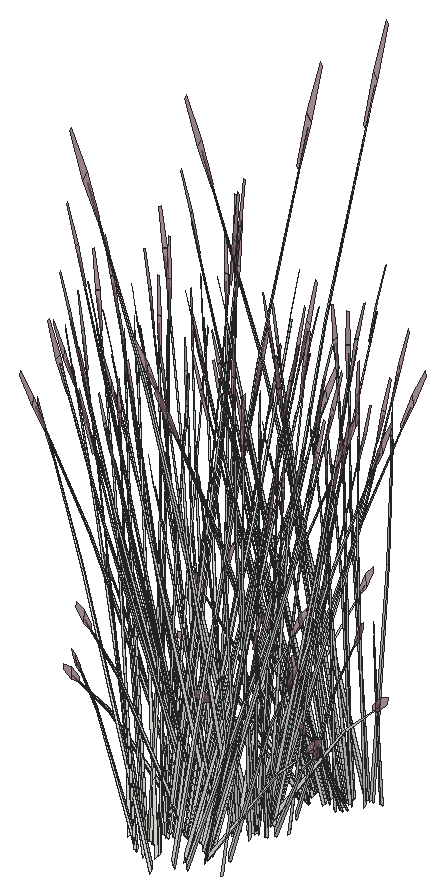
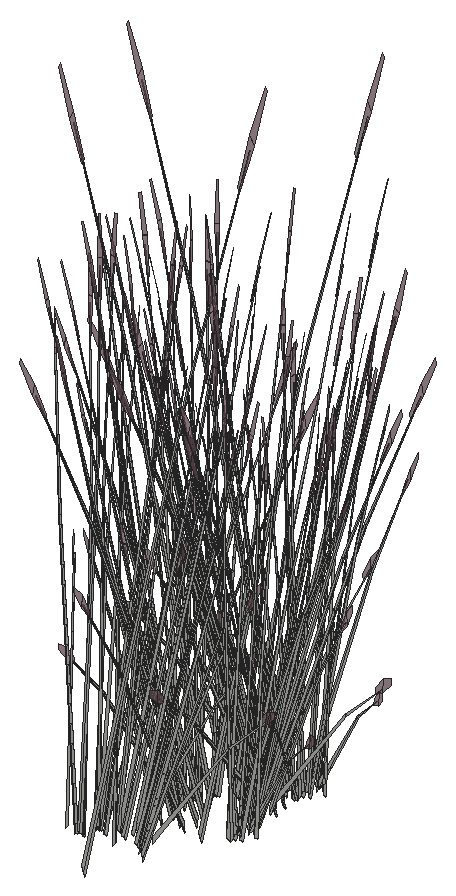
# SketchUp Ruby script. Lengths in inches.
U = 1.inch
M = Sketchup.active_model
def pt(a) = Geom::Point3d.new(a.map { |v| v * U })
def face(e, loops, mat)
  f = e.add_face(loops[0].map { |a| pt(a) })
  loops[1..].each { |l| e.add_face(l.map { |a| pt(a) }).erase! }
  f.material = f.back_material = mat if mat
  f
end
# faces: each face lists its corners as indices into pts; further lists are holes
def faces(e, pts, list, mat = nil) = list.each { |f| face(e, (f[0].is_a?(Array) ? f : [f]).map { |l| l.map { |i| pts[i] } }, mat) }
# xy, xz, yz: faces in a plane at the given z, y or x. An outline is a flat list of corners, or four numbers for a rectangle; further outlines are holes
def ring(l) = l.size == 4 ? [[l[0], l[1]], [l[2], l[1]], [l[2], l[3]], [l[0], l[3]]] : l.each_slice(2).to_a
def flat(e, list, mat, &to3) = list.each { |f| face(e, (f[0].is_a?(Array) ? f : [f]).map { |l| ring(l).map { |u, v| to3.(u, v) } }, mat) }
def xy(e, z, list, mat = nil) = flat(e, list, mat) { |x, y| [x, y, z] }
def xz(e, y, list, mat = nil) = flat(e, list, mat) { |x, z| [x, y, z] }
def yz(e, x, list, mat = nil) = flat(e, list, mat) { |y, z| [x, y, z] }
def lines(e, pts, list) = list.each { |a, b| e.add_line(pt(pts[a]), pt(pts[b])) }
# prism: a flat outline (further loops are holes) pulled along v
def prism(e, loops, v, mat = nil)
  f = face(e, loops, mat); d = Geom::Vector3d.new(v.map { |x| x * U })
  f.pushpull(f.normal.samedirection?(d) ? d.length : -d.length)
end
def box(e, o, s, mat = nil) = prism(e, [[o, [o[0] + s[0], o[1], o[2]], [o[0] + s[0], o[1] + s[1], o[2]], [o[0], o[1] + s[1], o[2]]]], [0, 0, s[2]], mat)
def at(x, y, z, deg = 0) = Geom::Transformation.translation(pt([x, y, z])) * Geom::Transformation.rotation(ORIGIN, Z_AXIS, deg.degrees)
def axes(o, x, y, z) = Geom::Transformation.new([*x, 0, *y, 0, *z, 0, *pt(o).to_a, 1])
def part(name) = M.definitions.add(name)
# library, detail: a bought-in or finely detailed component or shape, given as its bounding box
def library(name, o, s) = part(name).tap { |d| box(d.entities, o, s) }
def detail(e, o, s) = box(e.add_group.entities, o, s)
def put(e, d, t, mat = nil) = e.add_instance(d, t).tap { |i| i.material = mat if mat }
def group(e, t, mat = nil) = e.add_group.tap { |g| g.transformation = t; g.material = mat if mat }.entities
root = M.entities
M.materials.add("LightPink_Translucent").color = [144, 107, 117]
M.materials["LightPink_Translucent"].alpha = 0.75
c1 = part("blade")
p = [[2.15,0.21,22],[0,0.17,0],[0.09,0.45,0],[2.18,0.31,22],[2.29,0.31,22],[0.38,0.45,0],
  [2.48,0.24,33],[2.49,0.24,33],[2.48,0.22,33]]
faces(c1.entities,p,[[0,1,2,3],[4,5,2,3],[6,3,4,7],[8,0,3,6]])
c2 = part("seeds")
p = [[0.3,-0.1,1.38],[-0.01,-0.03,1.59],[-0.01,-0.03,0.03],[0.14,-0.07,-0.07],[0.29,-0.03,3],[0.15,0.01,3.11]]
faces(c2.entities,p,[[0,1,2,3],[1,0,4,5]],"LightPink_Translucent")
c3 = part("blade with seeds")
put(c3.entities,c1,at(0,0,0))
put(c3.entities,c2,axes([2.4,0.25,30.99],[1.5799,-0.05474,1.17369],[-0.12525,1.92788,0.29478],[-0.07173,-0.02425,1.56792]))
put(root,c3,axes([428.76,411.52,154],[0.15051,0.3216,0.05432],[-0.27447,0.15741,0.42765],[0.12099,-0.03106,0.65209]))
put(root,c3,axes([426.12,413.29,153.98],[-0.00765,0.05653,1.49853],[-0.37706,0.20517,-0.1416],[-0.11096,-0.10488,0.26519]))
put(root,c3,axes([427.18,414.53,154.25],[-0.40102,0.2196,-0.10273],[-0.19707,-0.38974,-0.57019],[-0.05291,-0.16424,0.8664]))
put(root,c3,axes([428.02,415.02,154.25],[-0.45039,-0.02337,-0.10273],[0.01231,-0.44247,-0.57019],[0.03129,-0.17041,0.8664]))
put(root,c3,axes([425.84,410.68,152.82],[0.11649,-0.06823,1.49584],[0.04017,0.47639,0.11706],[-0.25231,0.06321,0.53462]))
put(root,c3,axes([427.99,414.74,153.82],[0.27728,-0.24833,-0.29918],[0.26248,0.28355,0.38624],[0.03994,-0.14407,0.73904]))
put(root,c3,axes([427.17,414.36,154],[0.30197,-0.1603,0.05432],[0.1478,0.29231,0.42765],[-0.02916,-0.12885,0.65209]))
put(root,c3,axes([426.1,414.74,154.21],[-0.34944,-0.22798,-0.60019],[0.24834,-0.39949,0.07243],[-0.1266,-0.13612,0.84903]))
put(root,c3,axes([425.98,414.43,153.82],[-0.06329,-0.37991,-0.29918],[0.36182,-0.10032,0.38624],[-0.09718,-0.10887,0.73904]))
put(root,c3,axes([429.41,412.8,153.98],[-0.03706,-0.04129,1.49853],[0.08106,-0.44261,-0.1416],[0.14596,-0.02828,0.26519]))
put(root,c3,axes([424.59,411,153.98],[-0.06692,0.06124,1.47793],[0.00569,0.44742,-0.23373],[-0.15339,0.05818,0.11853]))
put(root,c3,axes([425.04,410.94,153.95],[-0.11102,0.42903,-0.43168],[-0.38064,-0.14706,-0.33437],[-0.15325,0.03934,0.82598]))
put(root,c3,axes([425.02,410.57,154.25],[0.20619,0.42709,-0.10273],[-0.36595,0.20988,-0.57019],[-0.15422,0.05635,0.8664]))
put(root,c3,axes([426.14,414.4,154],[0.18625,-0.29962,0.05432],[0.26523,0.17444,0.42765],[-0.08575,-0.09606,0.65209]))
put(root,c3,axes([429.09,412.43,153.32],[-0.07843,-0.39649,-0.0295],[0.37072,-0.09115,-0.13375],[0.07742,0.02514,0.44114]))
put(root,c3,axes([428.13,412.42,154.25],[0.02194,-0.47967,-0.10273],[0.41546,0.01311,-0.57019],[0.16001,0.03332,0.8664]))
put(root,c3,axes([425.21,414.99,153.27],[0.15222,0.08126,1.44779],[-0.31502,0.34091,0.11706],[-0.19634,-0.15379,0.61892]))
put(root,c3,axes([425.94,414.75,153.95],[-0.40438,0.11212,-0.43168],[-0.07074,-0.4246,-0.33437],[-0.10862,-0.12168,0.82598]))
put(root,c3,axes([426.22,414.37,154.59],[-0.2735,0.45217,-0.11506],[-0.39608,-0.2605,-0.63862],[-0.13768,-0.12775,0.97037]))
put(root,c3,axes([428.09,414.87,154],[0.33677,0.02198,0.05432],[-0.00923,0.33185,0.42765],[0.03524,-0.12712,0.65209]))
put(root,c3,axes([428.33,415.76,154.21],[0.21406,-0.37215,-0.60019],[0.37511,0.26448,0.07243],[0.12781,-0.13483,0.84903]))
put(root,c3,axes([428.32,415.59,153.95],[-0.10528,-0.43067,-0.43168],[0.39868,-0.07534,-0.33437],[0.11425,-0.11568,0.82598]))
put(root,c3,axes([428.49,412.13,153.98],[0.08791,-0.00798,1.47793],[0.24113,-0.36643,-0.23373],[0.15637,0.04837,0.11853]))
put(root,c3,axes([424.9,411.6875,154],[-0.28133,-0.19836,0.05432],[0.16379,-0.28248,0.42765],[-0.0902,0.09132,0.65209]))
put(root,c3,axes([425.02,411.16,153.27],[0.14219,-0.09977,1.44779],[0.11971,0.461,0.11706],[-0.22323,0.10419,0.61892]))
put(root,c3,axes([425.18,414.24,153.98],[-0.08817,-0.00333,1.47793],[-0.28072,0.33293,-0.23373],[-0.14978,-0.06803,0.11853]))
put(root,c3,axes([428.51,415.9,154.25],[-0.37908,-0.26007,-0.10273],[0.21839,-0.37663,-0.57019],[0.1071,-0.13092,0.8664]))
put(root,c3,axes([428.15,412.18,154.21],[0.40965,0.01136,-0.60019],[-0.02751,0.47821,0.07243],[0.17355,0.05047,0.84903]))
put(root,c3,axes([426.94,417.32,152.81],[0.35414,0.19019,1.27785],[-0.34693,0.40974,0.50532],[-0.1554,-0.24285,1.07126]))
put(root,c3,axes([429.44,415.78,153.98],[-0.05353,-0.00358,1.49853],[-0.22227,-0.38383,-0.1416],[0.08926,-0.1262,0.26519]))
put(root,c3,axes([423.85,411.45,153.98],[0.0523,0.01265,1.49853],[0.16179,0.41674,-0.1416],[-0.10706,0.10938,0.26519]))
put(root,c3,axes([428.4,412.38,153.82],[0.23317,0.29531,-0.29918],[-0.26625,0.27955,0.38624],[0.13527,0.04253,0.73904]))
put(root,c3,axes([428.28,412.5,154],[-0.02064,0.35866,0.05432],[-0.3116,-0.00983,0.42765],[0.11936,0.03753,0.65209]))
put(root,c3,axes([428.61,415.63,153.82],[0.35672,-0.06741,-0.29918],[0.09419,0.38534,0.38624],[0.10222,-0.1035,0.73904]))
put(root,c3,axes([424.93,411.85,153.82],[-0.35672,0.06741,-0.29918],[-0.09419,-0.38534,0.38624],[-0.10222,0.1035,0.73904]))
put(root,c3,axes([425.27,414.99,154],[0.02064,-0.35866,0.05432],[0.3116,0.00983,0.42765],[-0.11936,-0.03753,0.65209]))
put(root,c3,axes([425.15,415.1,153.82],[-0.23317,-0.29531,-0.29918],[0.26625,-0.27955,0.38624],[-0.13527,-0.04253,0.73904]))
put(root,c3,axes([427.56,411.625,153.27],[-0.15222,-0.08126,1.44779],[0.31502,-0.34091,0.11706],[0.19634,0.15379,0.61892]))
put(root,c3,axes([425.39,415.3,154.21],[-0.40965,-0.01136,-0.60019],[0.02751,-0.47821,0.07243],[-0.17355,-0.05047,0.84903]))
put(root,c3,axes([427.59,410.56,153.78],[-0.35411,-0.24507,1.16821],[0.37391,-0.38156,0.50405],[0.11425,0.22994,1.12919]))
put(root,c3,axes([425.04,411.59,154.25],[0.37908,0.26007,-0.10273],[-0.21839,0.37663,-0.57019],[-0.1071,0.13092,0.8664]))
put(root,c3,axes([427.3125,412.9375,154.25],[0.2442,-0.40372,-0.10273],[0.35364,0.23259,-0.57019],[0.12293,0.11406,0.8664]))
put(root,c3,axes([428.65,415.8,154],[0.28133,0.19836,0.05432],[-0.16379,0.28248,0.42765],[0.0902,-0.09132,0.65209]))
put(root,c3,axes([429.64,416.24,153.98],[0.05687,-0.07184,1.47793],[-0.07279,-0.44069,-0.23373],[0.14268,-0.08356,0.11853]))
put(root,c3,axes([425.55,411.47,153.27],[0.10236,-0.14492,1.44779],[0.25844,0.39118,0.11706],[-0.17726,0.17814,0.61892]))
put(root,c3,axes([425.22,411.9,153.95],[0.10528,0.43067,-0.43168],[-0.39868,0.07534,-0.33437],[-0.11425,0.11568,0.82598]))
put(root,c3,axes([424.84,414.52,153.98],[0.03038,0.04707,1.49853],[-0.14646,0.42312,-0.1416],[-0.14833,0.00306,0.26519]))
put(root,c3,axes([426.99,413.27,153.98],[0.00121,-0.0571,1.49853],[0.35119,-0.25193,-0.1416],[0.12199,0.08992,0.26519]))
put(root,c3,axes([425.45,412.62,154],[-0.33677,-0.02198,0.05432],[0.00923,-0.33185,0.42765],[-0.03524,0.12712,0.65209]))
put(root,c3,axes([427.6,412.74,153.95],[0.40438,-0.11212,-0.43168],[0.07074,0.4246,-0.33437],[0.10862,0.12168,0.82598]))
put(root,c3,axes([425.26,415.4,153.95],[-0.29757,0.31243,-0.43168],[-0.2606,-0.33005,-0.33437],[-0.15119,-0.04754,0.82598]))
put(root,c3,axes([425.41,415.07,154.25],[-0.02194,0.47967,-0.10273],[-0.41546,-0.01311,-0.57019],[-0.16001,-0.03332,0.8664]))
put(root,c3,axes([427.4,413.08,154],[-0.18625,0.29962,0.05432],[-0.26523,-0.17444,0.42765],[0.08575,0.09606,0.65209]))
put(root,c3,axes([428.52,416.91,154.25],[-0.20619,-0.42709,-0.10273],[0.36595,-0.20988,-0.57019],[0.15422,-0.05635,0.8664]))
put(root,c3,axes([428.5,416.54,153.95],[0.11102,-0.42903,-0.43168],[0.38064,0.14706,-0.33437],[0.15325,-0.03934,0.82598]))
put(root,c3,axes([424.88,415.73,153.27],[0.16998,-0.01068,1.44779],[-0.11276,0.46299,0.11706],[-0.24224,-0.02864,0.61892]))
put(root,c3,axes([425.47,411.83,153.27],[0.0763,-0.16212,1.44779],[0.3201,0.3355,0.11706],[-0.1444,0.2091,0.61892]))
put(root,c3,axes([428.43,416.7,154.21],[0.3601,-0.20831,-0.60019],[0.20068,0.4288,0.07243],[0.17399,-0.04871,0.84903]))
put(root,c3,axes([426.37,413.13,154],[-0.30197,0.1603,0.05432],[-0.1478,-0.29231,0.42765],[0.02916,0.12885,0.65209]))
put(root,c3,axes([425.56,412.74,153.82],[-0.27728,0.24833,-0.29918],[-0.26248,-0.28355,0.38624],[-0.03994,0.14407,0.73904]))
put(root,c3,axes([424.6,412.67,153.98],[-0.01019,0.09334,1.47793],[0.28908,0.3247,-0.23373],[-0.07568,0.15355,0.11853]))
put(root,c3,axes([425.53,412.46,154.56],[0.45039,0.02337,-0.11403],[-0.01231,0.44247,-0.63292],[-0.03129,0.17041,0.9617]))
put(root,c3,axes([426.36,412.95,154.25],[0.40102,-0.2196,-0.10273],[0.19707,0.38974,-0.57019],[0.05291,0.16424,0.8664]))
put(root,c3,axes([424.78,415.97,154],[-0.15051,-0.3216,0.05432],[0.27447,-0.15741,0.42765],[-0.12099,0.03106,0.65209]))
put(root,c3,axes([425.83,412.63,154.23],[0.29336,0.31691,-0.47917],[-0.3099,0.27755,-0.37115],[-0.04464,0.16102,0.91684]))
put(root,c3,axes([426.7,412.93,153.95],[0.40284,0.11824,-0.43168],[-0.13808,0.40538,-0.33437],[0.03694,0.16321,0.82598]))
put(root,c3,axes([426.93,412.1,153.27],[-0.09368,-0.15143,1.44779],[0.43286,-0.12749,0.11706],[0.09783,0.23774,0.61892]))
put(root,c3,axes([426.52,413.18,153.82],[-0.12355,0.36271,-0.29918],[-0.36044,-0.10579,0.38624],[0.03305,0.14603,0.73904]))
put(root,c3,axes([428.74,416.74,153.82],[0.34057,0.13158,-0.29918],[-0.09933,0.38387,0.38624],[0.13712,-0.0352,0.73904]))
put(root,c3,axes([425.74,412.48,154.51],[-0.01066,0.43628,-0.66621],[-0.44902,-0.0293,0.0804],[-0.04739,0.18483,0.94242]))
put(root,c3,axes([424.57,413.63,153.98],[0.04649,-0.02848,1.49853],[0.38427,0.18941,-0.1416],[-0.00903,0.15771,0.26519]))
put(root,c3,axes([424.73,416.13,153.82],[-0.34057,-0.13158,-0.29918],[0.09933,-0.38387,0.38624],[-0.13712,0.0352,0.73904]))
put(root,c3,axes([426.17,412.17,153.27],[-0.01003,-0.18103,1.44779],[0.43473,0.12009,0.11706],[-0.02689,0.25798,0.61892]))
put(root,c3,axes([428.2,420.67,153.27],[0.09368,0.15143,1.44779],[-0.43286,0.12749,0.11706],[-0.09783,-0.23774,0.61892]))
put(root,c3,axes([427.81,416.26,153.27],[-0.16998,0.01068,1.44779],[0.11276,-0.46299,0.11706],[0.24224,0.02864,0.61892]))
put(root,c3,axes([428.91,419.67,153.98],[-0.06268,-0.06613,1.47793],[-0.4183,0.04193,-0.23373],[-0.06676,-0.15817,0.11853]))
put(root,c3,axes([426.56,412.86,154.21],[0.19559,0.38351,-0.60019],[-0.40262,0.21373,0.07243],[0.04574,0.1853,0.84903]))
put(root,c3,axes([428.6875,416.9,154],[0.15051,0.3216,0.05432],[-0.27447,0.15741,0.42765],[0.12099,-0.03106,0.65209]))
put(root,c3,axes([426.26,413.83,153.98],[0.05195,0.07595,1.47793],[0.41921,0.02984,-0.23373],[0.04216,0.1675,0.11853]))
put(root,c3,axes([425.77,416.0625,152.82],[0.11649,-0.06823,1.49584],[0.04017,0.47639,0.11706],[-0.25231,0.06321,0.53462]))
put(root,c3,axes([430.79,420.48,153.98],[-0.00396,-0.09387,1.47793],[-0.33411,-0.2713,-0.23373],[0.05166,-0.16446,0.11853]))
put(root,c3,axes([429.39,420.46,153.82],[0.12355,-0.36271,-0.29918],[0.36044,0.10579,0.38624],[-0.03305,-0.14603,0.73904]))
put(root,c3,axes([429.66,420.9375,153.27],[-0.0763,0.16212,1.44779],[-0.3201,-0.3355,0.11706],[0.1444,-0.2091,0.61892]))
put(root,c3,axes([430.7,420.14,153.98],[-0.04162,0.03603,1.49853],[-0.40776,-0.12155,-0.1416],[-0.01476,-0.15722,0.26519]))
put(root,c3,axes([425.59,413.1,152.84],[0.009,-0.24349,1.30391],[0.40497,0.12861,0.18019],[-0.03509,0.2595,0.61571]))
put(root,c3,axes([429.21,420.71,153.95],[-0.40284,-0.11824,-0.43168],[0.13808,-0.40538,-0.33437],[-0.03694,-0.16321,0.82598]))
put(root,c3,axes([429.34,418.18,153.98],[-0.03706,-0.04129,1.49853],[0.08106,-0.44261,-0.1416],[0.14596,-0.02828,0.26519]))
put(root,c3,axes([430.08,421.01,153.95],[-0.29336,-0.31691,-0.43168],[0.3099,-0.27755,-0.33437],[0.04464,-0.16102,0.82598]))
put(root,c3,axes([424.52,416.38,153.98],[-0.06692,0.06124,1.47793],[0.00569,0.44742,-0.23373],[-0.15339,0.05818,0.11853]))
put(root,c3,axes([424.97,416.32,153.95],[-0.11102,0.42903,-0.43168],[-0.38064,-0.14706,-0.33437],[-0.15325,0.03934,0.82598]))
put(root,c3,axes([424.95,415.96,154.25],[0.20619,0.42709,-0.10273],[-0.36595,0.20988,-0.57019],[-0.15422,0.05635,0.8664]))
put(root,c3,axes([429.02,417.81,153.32],[-0.07843,-0.39649,-0.0295],[0.37072,-0.09115,-0.13375],[0.07742,0.02514,0.44114]))
put(root,c3,axes([428.49,419.45,153.98],[-0.00765,0.05653,1.49853],[-0.37706,0.20517,-0.1416],[-0.11096,-0.10488,0.26519]))
put(root,c3,axes([428.06,417.8,154.25],[0.02194,-0.47967,-0.10273],[0.41546,0.01311,-0.57019],[0.16001,0.03332,0.8664]))
put(root,c3,axes([429.43,420.54,154],[0.4038,0.12331,0.40553],[-0.13808,0.40538,0.33437],[-0.02427,-0.15942,0.83914]))
put(root,c3,axes([429.55,420.6875,154.25],[-0.40102,0.2196,-0.10273],[-0.19707,-0.38974,-0.57019],[-0.05291,-0.16424,0.8664]))
put(root,c3,axes([430.38,421.18,154.25],[-0.45039,-0.02337,-0.10273],[0.01231,-0.44247,-0.57019],[0.03129,-0.17041,0.8664]))
put(root,c3,axes([430.35,420.9,153.82],[0.27728,-0.24833,-0.29918],[0.26248,0.28355,0.38624],[0.03994,-0.14407,0.73904]))
put(root,c3,axes([429.54,420.51,154],[0.30197,-0.1603,0.05432],[0.1478,0.29231,0.42765],[-0.02916,-0.12885,0.65209]))
put(root,c3,axes([428.35,420.59,153.82],[-0.06329,-0.37991,-0.29918],[0.36182,-0.10032,0.38624],[-0.09718,-0.10887,0.73904]))
put(root,c3,axes([428.42,417.51,153.98],[0.08791,-0.00798,1.47793],[0.24113,-0.36643,-0.23373],[0.15637,0.04837,0.11853]))
put(root,c3,axes([424.83,417.07,154],[-0.28133,-0.19836,0.05432],[0.16379,-0.28248,0.42765],[-0.0902,0.09132,0.65209]))
put(root,c3,axes([424.95,416.54,153.27],[0.14219,-0.09977,1.44779],[0.11971,0.461,0.11706],[-0.22323,0.10419,0.61892]))
put(root,c3,axes([428.51,420.56,154],[0.18625,-0.29962,0.05432],[0.26523,0.17444,0.42765],[-0.08575,-0.09606,0.65209]))
put(root,c3,axes([427.57,421.14,153.27],[0.15222,0.08126,1.44779],[-0.31502,0.34091,0.11706],[-0.19634,-0.15379,0.61892]))
put(root,c3,axes([428.08,417.57,154.21],[0.40965,0.01136,-0.60019],[-0.02751,0.47821,0.07243],[0.17355,0.05047,0.84903]))
put(root,c3,axes([428.31,420.9,153.95],[-0.40438,0.11212,-0.43168],[-0.07074,-0.4246,-0.33437],[-0.10862,-0.12168,0.82598]))
put(root,c3,axes([430.35,420.99,154],[0.29182,0.32181,0.40553],[-0.3099,0.27755,0.33437],[0.05383,-0.15098,0.83914]))
put(root,c3,axes([428.59,420.52,154.59],[-0.2735,0.45217,-0.11506],[-0.39608,-0.2605,-0.63862],[-0.13768,-0.12775,0.97037]))
put(root,c3,axes([430.46,421.02,154],[0.33677,0.02198,0.05432],[-0.00923,0.33185,0.42765],[0.03524,-0.12712,0.65209]))
put(root,c3,axes([423.78,416.84,153.98],[0.0523,0.01265,1.49853],[0.16179,0.41674,-0.1416],[-0.10706,0.10938,0.26519]))
put(root,c3,axes([430.6875,421.74,153.95],[-0.10528,-0.43067,-0.43168],[0.39868,-0.07534,-0.33437],[0.11425,-0.11568,0.82598]))
put(root,c3,axes([428.33,417.76,153.82],[0.23317,0.29531,-0.29918],[-0.26625,0.27955,0.38624],[0.13527,0.04253,0.73904]))
put(root,c3,axes([428.21,417.88,154],[-0.02064,0.35866,0.05432],[-0.3116,-0.00983,0.42765],[0.11936,0.03753,0.65209]))
put(root,c3,axes([424.86,417.23,153.82],[-0.35672,0.06741,-0.29918],[-0.09419,-0.38534,0.38624],[-0.10222,0.1035,0.73904]))
put(root,c3,axes([427.54,420.39,153.98],[-0.08817,-0.00333,1.47793],[-0.28072,0.33293,-0.23373],[-0.14978,-0.06803,0.11853]))
put(root,c3,axes([430.875,422.05,154.25],[-0.37908,-0.26007,-0.10273],[0.21839,-0.37663,-0.57019],[0.1071,-0.13092,0.8664]))
put(root,c3,axes([429.31,423.47,152.81],[0.35414,0.19019,1.27785],[-0.34693,0.40974,0.50532],[-0.1554,-0.24285,1.07126]))
put(root,c3,axes([431.81,421.9375,153.98],[-0.05353,-0.00358,1.49853],[-0.22227,-0.38383,-0.1416],[0.08926,-0.1262,0.26519]))
put(root,c3,axes([427.49,417.01,153.27],[-0.15222,-0.08126,1.44779],[0.31502,-0.34091,0.11706],[0.19634,0.15379,0.61892]))
put(root,c3,axes([427.52,415.9375,153.78],[-0.35411,-0.24507,1.16821],[0.37391,-0.38156,0.50405],[0.11425,0.22994,1.12919]))
put(root,c3,axes([424.97,416.97,154.25],[0.37908,0.26007,-0.10273],[-0.21839,0.37663,-0.57019],[-0.1071,0.13092,0.8664]))
put(root,c3,axes([427.24,418.32,154.25],[0.2442,-0.40372,-0.10273],[0.35364,0.23259,-0.57019],[0.12293,0.11406,0.8664]))
put(root,c3,axes([430.98,421.79,153.82],[0.35672,-0.06741,-0.29918],[0.09419,0.38534,0.38624],[0.10222,-0.1035,0.73904]))
put(root,c3,axes([427.63,421.15,154],[0.02064,-0.35866,0.05432],[0.3116,0.00983,0.42765],[-0.11936,-0.03753,0.65209]))
put(root,c3,axes([425.48,416.86,153.27],[0.10236,-0.14492,1.44779],[0.25844,0.39118,0.11706],[-0.17726,0.17814,0.61892]))
put(root,c3,axes([427.51,421.26,153.82],[-0.23317,-0.29531,-0.29918],[0.26625,-0.27955,0.38624],[-0.13527,-0.04253,0.73904]))
put(root,c3,axes([425.15,417.28,153.95],[0.10528,0.43067,-0.43168],[-0.39868,0.07534,-0.33437],[-0.11425,0.11568,0.82598]))
put(root,c3,axes([426.92,418.65,153.98],[0.00121,-0.0571,1.49853],[0.35119,-0.25193,-0.1416],[0.12199,0.08992,0.26519]))
